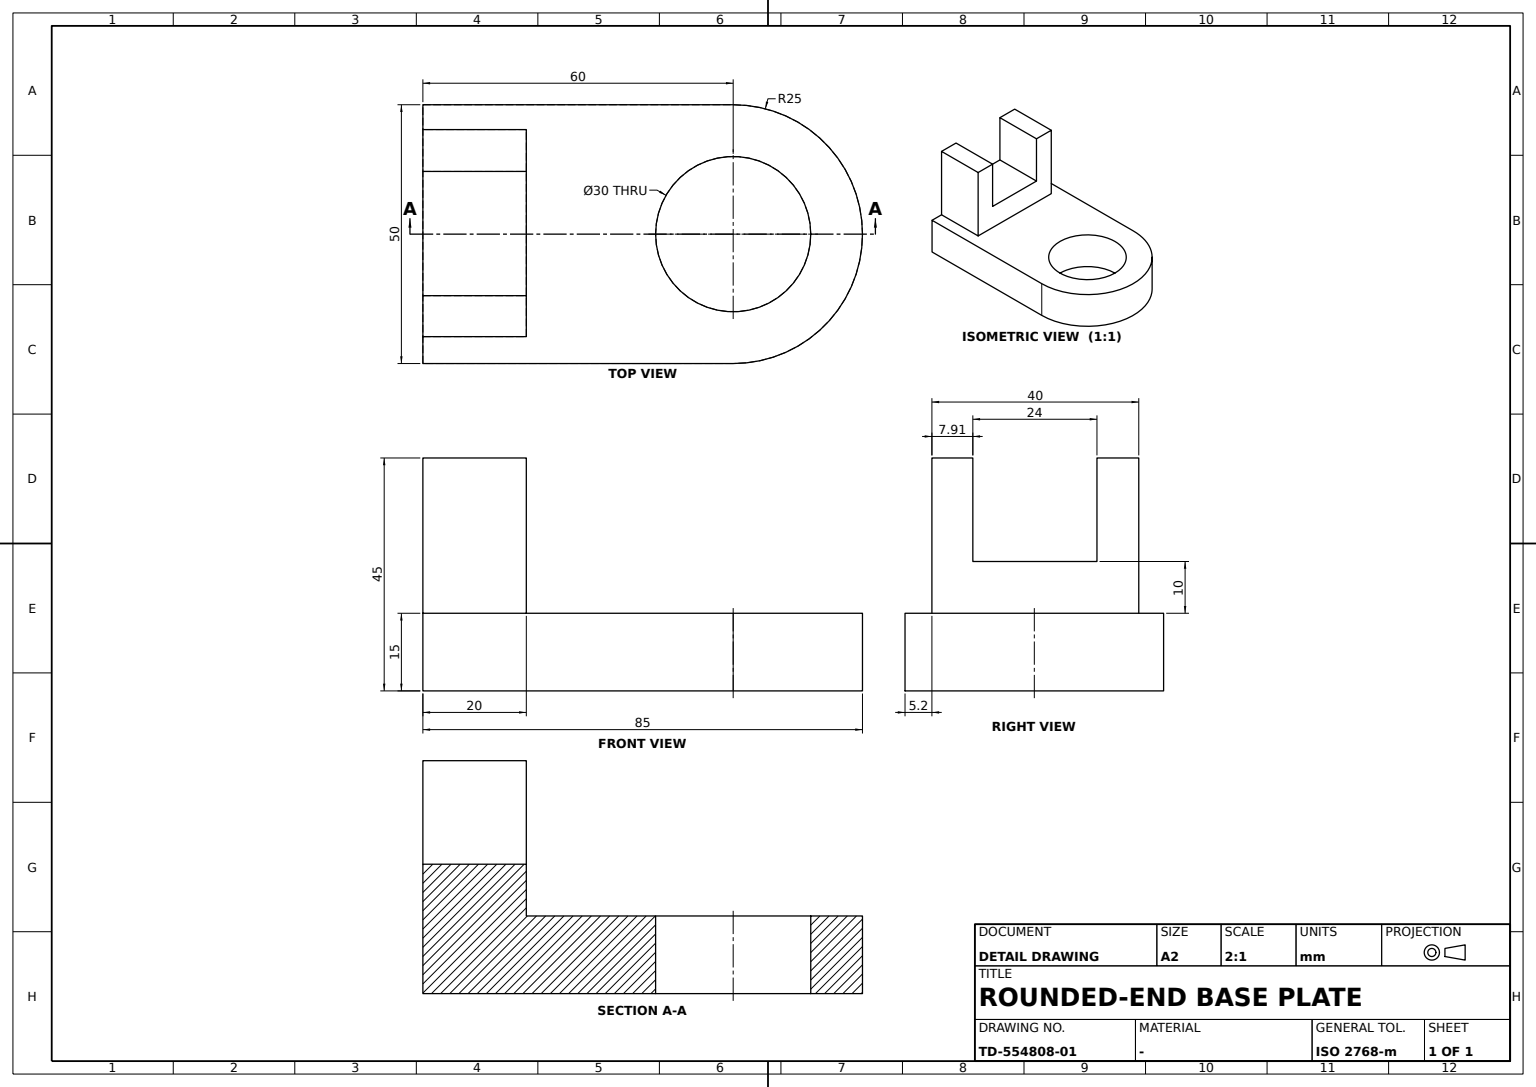
ISO-10303-21;
HEADER;
FILE_DESCRIPTION((''),'2;1');
FILE_NAME('','',(''),(''),'','','');
FILE_SCHEMA(('AUTOMOTIVE_DESIGN'));
ENDSEC;
DATA;
#1=APPLICATION_CONTEXT('');
#2=PRODUCT_CONTEXT('',#1,'mechanical');
#3=PRODUCT('','','',(#2));
#4=PRODUCT_DEFINITION_FORMATION('','',#3);
#5=PRODUCT_DEFINITION_CONTEXT('',#1,'design');
#6=PRODUCT_DEFINITION('','',#4,#5);
#7=PRODUCT_DEFINITION_SHAPE('','',#6);
#8=(LENGTH_UNIT()NAMED_UNIT(*)SI_UNIT(.MILLI.,.METRE.));
#9=(NAMED_UNIT(*)PLANE_ANGLE_UNIT()SI_UNIT($,.RADIAN.));
#10=(NAMED_UNIT(*)SI_UNIT($,.STERADIAN.)SOLID_ANGLE_UNIT());
#11=UNCERTAINTY_MEASURE_WITH_UNIT(LENGTH_MEASURE(0.005),#8,'distance_accuracy_value','');
#12=(GEOMETRIC_REPRESENTATION_CONTEXT(3)GLOBAL_UNCERTAINTY_ASSIGNED_CONTEXT((#11))GLOBAL_UNIT_ASSIGNED_CONTEXT((#8,#9,#10))REPRESENTATION_CONTEXT('',''));
#13=CARTESIAN_POINT('',(0.,-25.,0.));
#14=VERTEX_POINT('',#13);
#15=CARTESIAN_POINT('',(0.,25.,0.));
#16=VERTEX_POINT('',#15);
#17=CARTESIAN_POINT('',(0.,0.,0.));
#18=DIRECTION('',(0.,0.,1.));
#19=DIRECTION('',(1.,0.,0.));
#20=AXIS2_PLACEMENT_3D('',#17,#18,#19);
#21=CIRCLE('',#20,25.);
#22=EDGE_CURVE('',#14,#16,#21,.T.);
#23=ORIENTED_EDGE('',*,*,#22,.T.);
#24=CARTESIAN_POINT('',(0.,25.,15.));
#25=VERTEX_POINT('',#24);
#26=CARTESIAN_POINT('',(0.,25.,7.5));
#27=VECTOR('',#18,1000.);
#28=LINE('',#26,#27);
#29=EDGE_CURVE('',#16,#25,#28,.T.);
#30=ORIENTED_EDGE('',*,*,#29,.T.);
#31=CARTESIAN_POINT('',(0.,-25.,15.));
#32=VERTEX_POINT('',#31);
#33=CARTESIAN_POINT('',(0.,0.,15.));
#34=AXIS2_PLACEMENT_3D('',#33,#18,#19);
#35=CIRCLE('',#34,25.);
#36=EDGE_CURVE('',#32,#25,#35,.T.);
#37=ORIENTED_EDGE('',*,*,#36,.F.);
#38=CARTESIAN_POINT('',(0.,-25.,7.5));
#39=LINE('',#38,#27);
#40=EDGE_CURVE('',#14,#32,#39,.T.);
#41=ORIENTED_EDGE('',*,*,#40,.F.);
#42=EDGE_LOOP('',(#23,#30,#37,#41));
#43=FACE_BOUND('',#42,.T.);
#44=CARTESIAN_POINT('',(0.,0.,7.5));
#45=DIRECTION('',(0.,1.,0.));
#46=AXIS2_PLACEMENT_3D('',#44,#18,#45);
#47=CYLINDRICAL_SURFACE('',#46,25.);
#48=ADVANCED_FACE('',(#43),#47,.T.);
#49=CARTESIAN_POINT('',(-60.,-25.,15.));
#50=VERTEX_POINT('',#49);
#51=CARTESIAN_POINT('',(-60.,-19.801716,15.));
#52=VERTEX_POINT('',#51);
#53=CARTESIAN_POINT('',(-60.,0.,15.));
#54=VECTOR('',#45,1000.);
#55=LINE('',#53,#54);
#56=EDGE_CURVE('',#50,#52,#55,.T.);
#57=ORIENTED_EDGE('',*,*,#56,.T.);
#58=CARTESIAN_POINT('',(-60.,-19.801716,45.));
#59=VERTEX_POINT('',#58);
#60=CARTESIAN_POINT('',(-60.,-19.801716,0.));
#61=LINE('',#60,#27);
#62=EDGE_CURVE('',#52,#59,#61,.T.);
#63=ORIENTED_EDGE('',*,*,#62,.T.);
#64=CARTESIAN_POINT('',(-60.,-11.887171,45.));
#65=VERTEX_POINT('',#64);
#66=CARTESIAN_POINT('',(-60.,-25.,45.));
#67=LINE('',#66,#54);
#68=EDGE_CURVE('',#59,#65,#67,.T.);
#69=ORIENTED_EDGE('',*,*,#68,.T.);
#70=CARTESIAN_POINT('',(-60.,-11.887171,25.));
#71=VERTEX_POINT('',#70);
#72=CARTESIAN_POINT('',(-60.,-11.887171,0.));
#73=DIRECTION('',(0.,0.,-1.));
#74=VECTOR('',#73,1000.);
#75=LINE('',#72,#74);
#76=EDGE_CURVE('',#65,#71,#75,.T.);
#77=ORIENTED_EDGE('',*,*,#76,.T.);
#78=CARTESIAN_POINT('',(-60.,12.112829,25.));
#79=VERTEX_POINT('',#78);
#80=CARTESIAN_POINT('',(-60.,-25.,25.));
#81=LINE('',#80,#54);
#82=EDGE_CURVE('',#71,#79,#81,.T.);
#83=ORIENTED_EDGE('',*,*,#82,.T.);
#84=CARTESIAN_POINT('',(-60.,12.112829,45.));
#85=VERTEX_POINT('',#84);
#86=CARTESIAN_POINT('',(-60.,12.112829,0.));
#87=LINE('',#86,#27);
#88=EDGE_CURVE('',#79,#85,#87,.T.);
#89=ORIENTED_EDGE('',*,*,#88,.T.);
#90=CARTESIAN_POINT('',(-60.,20.198284,45.));
#91=VERTEX_POINT('',#90);
#92=EDGE_CURVE('',#85,#91,#67,.T.);
#93=ORIENTED_EDGE('',*,*,#92,.T.);
#94=CARTESIAN_POINT('',(-60.,20.198284,15.));
#95=VERTEX_POINT('',#94);
#96=CARTESIAN_POINT('',(-60.,20.198284,0.));
#97=LINE('',#96,#74);
#98=EDGE_CURVE('',#91,#95,#97,.T.);
#99=ORIENTED_EDGE('',*,*,#98,.T.);
#100=CARTESIAN_POINT('',(-60.,25.,15.));
#101=VERTEX_POINT('',#100);
#102=EDGE_CURVE('',#95,#101,#55,.T.);
#103=ORIENTED_EDGE('',*,*,#102,.T.);
#104=CARTESIAN_POINT('',(-60.,25.,0.));
#105=VERTEX_POINT('',#104);
#106=LINE('',#104,#27);
#107=EDGE_CURVE('',#105,#101,#106,.T.);
#108=ORIENTED_EDGE('',*,*,#107,.F.);
#109=CARTESIAN_POINT('',(-60.,-25.,0.));
#110=VERTEX_POINT('',#109);
#111=CARTESIAN_POINT('',(-60.,0.,0.));
#112=LINE('',#111,#54);
#113=EDGE_CURVE('',#110,#105,#112,.T.);
#114=ORIENTED_EDGE('',*,*,#113,.F.);
#115=LINE('',#109,#27);
#116=EDGE_CURVE('',#110,#50,#115,.T.);
#117=ORIENTED_EDGE('',*,*,#116,.T.);
#118=EDGE_LOOP('',(#57,#63,#69,#77,#83,#89,#93,#99,#103,#108,#114,#117));
#119=FACE_BOUND('',#118,.T.);
#120=AXIS2_PLACEMENT_3D('',#109,#19,#45);
#121=PLANE('',#120);
#122=ADVANCED_FACE('',(#119),#121,.F.);
#123=ORIENTED_EDGE('',*,*,#88,.F.);
#124=CARTESIAN_POINT('',(-40.,12.112829,25.));
#125=VERTEX_POINT('',#124);
#126=VECTOR('',#19,1000.);
#127=LINE('',#78,#126);
#128=EDGE_CURVE('',#79,#125,#127,.T.);
#129=ORIENTED_EDGE('',*,*,#128,.T.);
#130=CARTESIAN_POINT('',(-40.,12.112829,45.));
#131=VERTEX_POINT('',#130);
#132=LINE('',#124,#27);
#133=EDGE_CURVE('',#125,#131,#132,.T.);
#134=ORIENTED_EDGE('',*,*,#133,.T.);
#135=LINE('',#84,#126);
#136=EDGE_CURVE('',#85,#131,#135,.T.);
#137=ORIENTED_EDGE('',*,*,#136,.F.);
#138=EDGE_LOOP('',(#123,#129,#134,#137));
#139=FACE_BOUND('',#138,.T.);
#140=AXIS2_PLACEMENT_3D('',#78,#45,#18);
#141=PLANE('',#140);
#142=ADVANCED_FACE('',(#139),#141,.F.);
#143=CARTESIAN_POINT('',(-40.,-19.801716,15.));
#144=VERTEX_POINT('',#143);
#145=CARTESIAN_POINT('',(-40.,-19.801716,45.));
#146=VERTEX_POINT('',#145);
#147=LINE('',#143,#27);
#148=EDGE_CURVE('',#144,#146,#147,.T.);
#149=ORIENTED_EDGE('',*,*,#148,.T.);
#150=LINE('',#58,#126);
#151=EDGE_CURVE('',#59,#146,#150,.T.);
#152=ORIENTED_EDGE('',*,*,#151,.F.);
#153=ORIENTED_EDGE('',*,*,#62,.F.);
#154=LINE('',#51,#126);
#155=EDGE_CURVE('',#52,#144,#154,.T.);
#156=ORIENTED_EDGE('',*,*,#155,.T.);
#157=EDGE_LOOP('',(#149,#152,#153,#156));
#158=FACE_BOUND('',#157,.T.);
#159=AXIS2_PLACEMENT_3D('',#51,#45,#18);
#160=PLANE('',#159);
#161=ADVANCED_FACE('',(#158),#160,.F.);
#162=DIRECTION('',(-1.,0.,0.));
#163=VECTOR('',#162,1000.);
#164=LINE('',#13,#163);
#165=EDGE_CURVE('',#14,#110,#164,.T.);
#166=ORIENTED_EDGE('',*,*,#165,.T.);
#167=ORIENTED_EDGE('',*,*,#113,.T.);
#168=LINE('',#15,#163);
#169=EDGE_CURVE('',#16,#105,#168,.T.);
#170=ORIENTED_EDGE('',*,*,#169,.F.);
#171=ORIENTED_EDGE('',*,*,#22,.F.);
#172=EDGE_LOOP('',(#166,#167,#170,#171));
#173=FACE_BOUND('',#172,.T.);
#174=CARTESIAN_POINT('',(15.,0.,0.));
#175=VERTEX_POINT('',#174);
#176=CIRCLE('',#20,15.);
#177=EDGE_CURVE('',#175,#175,#176,.T.);
#178=ORIENTED_EDGE('',*,*,#177,.T.);
#179=EDGE_LOOP('',(#178));
#180=FACE_BOUND('',#179,.T.);
#181=AXIS2_PLACEMENT_3D('',#17,#18,#45);
#182=PLANE('',#181);
#183=ADVANCED_FACE('',(#173,#180),#182,.F.);
#184=ORIENTED_EDGE('',*,*,#76,.F.);
#185=CARTESIAN_POINT('',(-40.,-11.887171,45.));
#186=VERTEX_POINT('',#185);
#187=LINE('',#64,#126);
#188=EDGE_CURVE('',#65,#186,#187,.T.);
#189=ORIENTED_EDGE('',*,*,#188,.T.);
#190=CARTESIAN_POINT('',(-40.,-11.887171,25.));
#191=VERTEX_POINT('',#190);
#192=LINE('',#185,#74);
#193=EDGE_CURVE('',#186,#191,#192,.T.);
#194=ORIENTED_EDGE('',*,*,#193,.T.);
#195=LINE('',#70,#126);
#196=EDGE_CURVE('',#71,#191,#195,.T.);
#197=ORIENTED_EDGE('',*,*,#196,.F.);
#198=EDGE_LOOP('',(#184,#189,#194,#197));
#199=FACE_BOUND('',#198,.T.);
#200=DIRECTION('',(0.,-1.,0.));
#201=AXIS2_PLACEMENT_3D('',#64,#200,#73);
#202=PLANE('',#201);
#203=ADVANCED_FACE('',(#199),#202,.F.);
#204=ORIENTED_EDGE('',*,*,#165,.F.);
#205=ORIENTED_EDGE('',*,*,#40,.T.);
#206=LINE('',#31,#163);
#207=EDGE_CURVE('',#32,#50,#206,.T.);
#208=ORIENTED_EDGE('',*,*,#207,.T.);
#209=ORIENTED_EDGE('',*,*,#116,.F.);
#210=EDGE_LOOP('',(#204,#205,#208,#209));
#211=FACE_BOUND('',#210,.T.);
#212=AXIS2_PLACEMENT_3D('',#13,#45,#162);
#213=PLANE('',#212);
#214=ADVANCED_FACE('',(#211),#213,.F.);
#215=ORIENTED_EDGE('',*,*,#196,.T.);
#216=LINE('',#190,#54);
#217=EDGE_CURVE('',#191,#125,#216,.T.);
#218=ORIENTED_EDGE('',*,*,#217,.T.);
#219=ORIENTED_EDGE('',*,*,#128,.F.);
#220=ORIENTED_EDGE('',*,*,#82,.F.);
#221=EDGE_LOOP('',(#215,#218,#219,#220));
#222=FACE_BOUND('',#221,.T.);
#223=AXIS2_PLACEMENT_3D('',#70,#73,#45);
#224=PLANE('',#223);
#225=ADVANCED_FACE('',(#222),#224,.F.);
#226=CARTESIAN_POINT('',(15.,0.,15.));
#227=VERTEX_POINT('',#226);
#228=CIRCLE('',#34,15.);
#229=EDGE_CURVE('',#227,#227,#228,.T.);
#230=ORIENTED_EDGE('',*,*,#229,.F.);
#231=EDGE_LOOP('',(#230));
#232=FACE_BOUND('',#231,.T.);
#233=ORIENTED_EDGE('',*,*,#36,.T.);
#234=LINE('',#24,#163);
#235=EDGE_CURVE('',#25,#101,#234,.T.);
#236=ORIENTED_EDGE('',*,*,#235,.T.);
#237=ORIENTED_EDGE('',*,*,#102,.F.);
#238=CARTESIAN_POINT('',(-40.,20.198284,15.));
#239=VERTEX_POINT('',#238);
#240=CARTESIAN_POINT('',(0.,20.198284,15.));
#241=LINE('',#240,#126);
#242=EDGE_CURVE('',#95,#239,#241,.T.);
#243=ORIENTED_EDGE('',*,*,#242,.T.);
#244=CARTESIAN_POINT('',(-40.,0.,15.));
#245=VECTOR('',#200,1000.);
#246=LINE('',#244,#245);
#247=EDGE_CURVE('',#239,#144,#246,.T.);
#248=ORIENTED_EDGE('',*,*,#247,.T.);
#249=ORIENTED_EDGE('',*,*,#155,.F.);
#250=ORIENTED_EDGE('',*,*,#56,.F.);
#251=ORIENTED_EDGE('',*,*,#207,.F.);
#252=EDGE_LOOP('',(#233,#236,#237,#243,#248,#249,#250,#251));
#253=FACE_BOUND('',#252,.T.);
#254=AXIS2_PLACEMENT_3D('',#33,#18,#45);
#255=PLANE('',#254);
#256=ADVANCED_FACE('',(#232,#253),#255,.T.);
#257=ORIENTED_EDGE('',*,*,#177,.F.);
#258=EDGE_LOOP('',(#257));
#259=FACE_BOUND('',#258,.T.);
#260=ORIENTED_EDGE('',*,*,#229,.T.);
#261=EDGE_LOOP('',(#260));
#262=FACE_BOUND('',#261,.T.);
#263=CARTESIAN_POINT('',(0.,0.,14.9));
#264=AXIS2_PLACEMENT_3D('',#263,#73,#19);
#265=CYLINDRICAL_SURFACE('',#264,15.);
#266=ADVANCED_FACE('',(#259,#262),#265,.F.);
#267=ORIENTED_EDGE('',*,*,#242,.F.);
#268=ORIENTED_EDGE('',*,*,#98,.F.);
#269=CARTESIAN_POINT('',(-40.,20.198284,45.));
#270=VERTEX_POINT('',#269);
#271=LINE('',#90,#126);
#272=EDGE_CURVE('',#91,#270,#271,.T.);
#273=ORIENTED_EDGE('',*,*,#272,.T.);
#274=LINE('',#269,#74);
#275=EDGE_CURVE('',#270,#239,#274,.T.);
#276=ORIENTED_EDGE('',*,*,#275,.T.);
#277=EDGE_LOOP('',(#267,#268,#273,#276));
#278=FACE_BOUND('',#277,.T.);
#279=AXIS2_PLACEMENT_3D('',#90,#200,#73);
#280=PLANE('',#279);
#281=ADVANCED_FACE('',(#278),#280,.F.);
#282=ORIENTED_EDGE('',*,*,#68,.F.);
#283=ORIENTED_EDGE('',*,*,#151,.T.);
#284=LINE('',#145,#54);
#285=EDGE_CURVE('',#146,#186,#284,.T.);
#286=ORIENTED_EDGE('',*,*,#285,.T.);
#287=ORIENTED_EDGE('',*,*,#188,.F.);
#288=EDGE_LOOP('',(#282,#283,#286,#287));
#289=FACE_BOUND('',#288,.T.);
#290=AXIS2_PLACEMENT_3D('',#58,#73,#45);
#291=PLANE('',#290);
#292=ADVANCED_FACE('',(#289),#291,.F.);
#293=ORIENTED_EDGE('',*,*,#29,.F.);
#294=ORIENTED_EDGE('',*,*,#169,.T.);
#295=ORIENTED_EDGE('',*,*,#107,.T.);
#296=ORIENTED_EDGE('',*,*,#235,.F.);
#297=EDGE_LOOP('',(#293,#294,#295,#296));
#298=FACE_BOUND('',#297,.T.);
#299=AXIS2_PLACEMENT_3D('',#15,#45,#162);
#300=PLANE('',#299);
#301=ADVANCED_FACE('',(#298),#300,.T.);
#302=ORIENTED_EDGE('',*,*,#92,.F.);
#303=ORIENTED_EDGE('',*,*,#136,.T.);
#304=EDGE_CURVE('',#131,#270,#284,.T.);
#305=ORIENTED_EDGE('',*,*,#304,.T.);
#306=ORIENTED_EDGE('',*,*,#272,.F.);
#307=EDGE_LOOP('',(#302,#303,#305,#306));
#308=FACE_BOUND('',#307,.T.);
#309=ADVANCED_FACE('',(#308),#291,.F.);
#310=ORIENTED_EDGE('',*,*,#304,.F.);
#311=ORIENTED_EDGE('',*,*,#133,.F.);
#312=ORIENTED_EDGE('',*,*,#217,.F.);
#313=ORIENTED_EDGE('',*,*,#193,.F.);
#314=ORIENTED_EDGE('',*,*,#285,.F.);
#315=ORIENTED_EDGE('',*,*,#148,.F.);
#316=ORIENTED_EDGE('',*,*,#247,.F.);
#317=ORIENTED_EDGE('',*,*,#275,.F.);
#318=EDGE_LOOP('',(#310,#311,#312,#313,#314,#315,#316,#317));
#319=FACE_BOUND('',#318,.T.);
#320=CARTESIAN_POINT('',(-40.,0.,0.));
#321=AXIS2_PLACEMENT_3D('',#320,#162,#200);
#322=PLANE('',#321);
#323=ADVANCED_FACE('',(#319),#322,.F.);
#324=CLOSED_SHELL('',(#48,#122,#142,#161,#183,#203,#214,#225,#256,#266,#281,#292,#301,#309,#323));
#325=MANIFOLD_SOLID_BREP('',#324);
#326=ADVANCED_BREP_SHAPE_REPRESENTATION('',(#325),#12);
#327=SHAPE_DEFINITION_REPRESENTATION(#7,#326);
ENDSEC;
END-ISO-10303-21;
